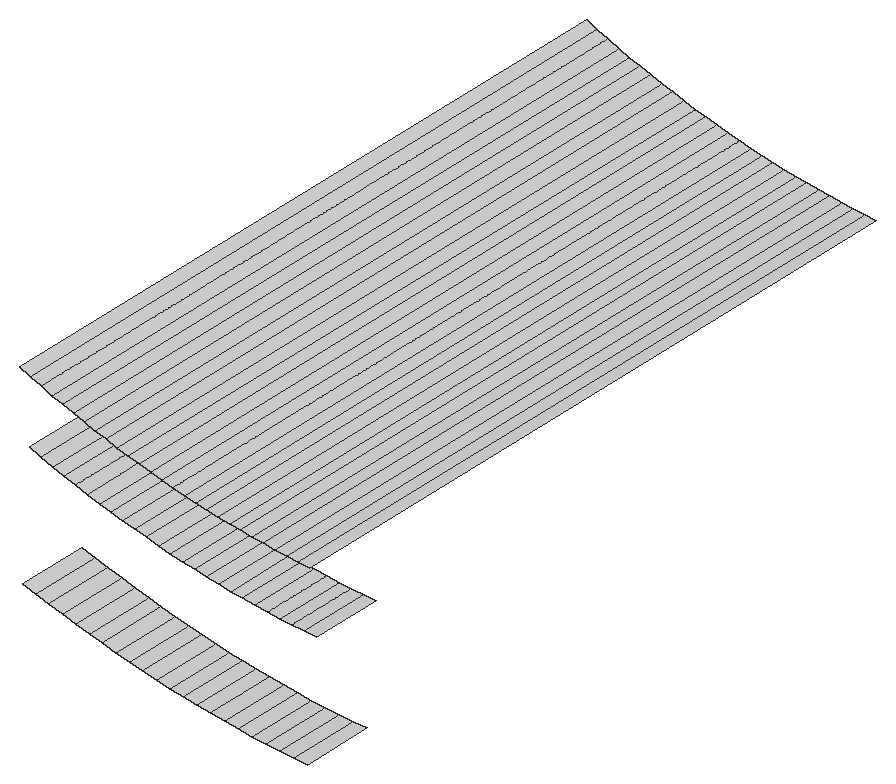
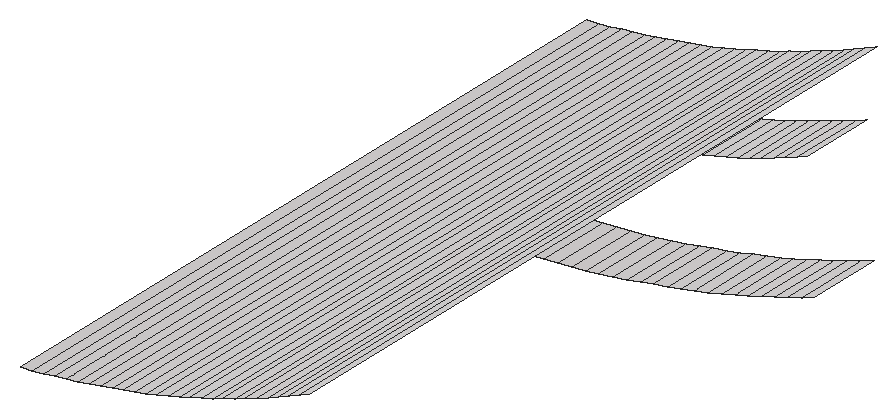
# SketchUp Ruby script. Lengths in inches.
U = 1.inch
M = Sketchup.active_model
def pt(a) = Geom::Point3d.new(a.map { |v| v * U })
def face(e, loops, mat)
  f = e.add_face(loops[0].map { |a| pt(a) })
  loops[1..].each { |l| e.add_face(l.map { |a| pt(a) }).erase! }
  f.material = f.back_material = mat if mat
  f
end
# faces: each face lists its corners as indices into pts; further lists are holes
def faces(e, pts, list, mat = nil) = list.each { |f| face(e, (f[0].is_a?(Array) ? f : [f]).map { |l| l.map { |i| pts[i] } }, mat) }
# xy, xz, yz: faces in a plane at the given z, y or x. An outline is a flat list of corners, or four numbers for a rectangle; further outlines are holes
def ring(l) = l.size == 4 ? [[l[0], l[1]], [l[2], l[1]], [l[2], l[3]], [l[0], l[3]]] : l.each_slice(2).to_a
def flat(e, list, mat, &to3) = list.each { |f| face(e, (f[0].is_a?(Array) ? f : [f]).map { |l| ring(l).map { |u, v| to3.(u, v) } }, mat) }
def xy(e, z, list, mat = nil) = flat(e, list, mat) { |x, y| [x, y, z] }
def xz(e, y, list, mat = nil) = flat(e, list, mat) { |x, z| [x, y, z] }
def yz(e, x, list, mat = nil) = flat(e, list, mat) { |y, z| [x, y, z] }
def lines(e, pts, list) = list.each { |a, b| e.add_line(pt(pts[a]), pt(pts[b])) }
# prism: a flat outline (further loops are holes) pulled along v
def prism(e, loops, v, mat = nil)
  f = face(e, loops, mat); d = Geom::Vector3d.new(v.map { |x| x * U })
  f.pushpull(f.normal.samedirection?(d) ? d.length : -d.length)
end
def box(e, o, s, mat = nil) = prism(e, [[o, [o[0] + s[0], o[1], o[2]], [o[0] + s[0], o[1] + s[1], o[2]], [o[0], o[1] + s[1], o[2]]]], [0, 0, s[2]], mat)
def at(x, y, z, deg = 0) = Geom::Transformation.translation(pt([x, y, z])) * Geom::Transformation.rotation(ORIGIN, Z_AXIS, deg.degrees)
def axes(o, x, y, z) = Geom::Transformation.new([*x, 0, *y, 0, *z, 0, *pt(o).to_a, 1])
def part(name) = M.definitions.add(name)
# library, detail: a bought-in or finely detailed component or shape, given as its bounding box
def library(name, o, s) = part(name).tap { |d| box(d.entities, o, s) }
def detail(e, o, s) = box(e.add_group.entities, o, s)
def put(e, d, t, mat = nil) = e.add_instance(d, t).tap { |i| i.material = mat if mat }
def group(e, t, mat = nil) = e.add_group.tap { |g| g.transformation = t; g.material = mat if mat }.entities
root = M.entities
M.materials.add("[Quartz Light Brown]").color = [215, 212, 212]
p = [[291.15,144.25,150.15],[291.15,143,150.15],[291.38,143,150.125],[291.38,144.25,150.125],[291.62,143,150.1],[291.62,144.25,150.1],
  [291.85,143,150.08],[291.85,144.25,150.08],[292.09,143,150.06],[292.09,144.25,150.06],[290.45,144.25,150.26],[290.45,143,150.26],
  [290.68,143,150.22],[290.68,144.25,150.22],[290.92,143,150.1875],[290.92,144.25,150.1875],[289.76,144.25,150.39],[289.76,143,150.39],
  [289.99,143,150.35],[289.99,144.25,150.35],[290.22,143,150.3],[290.22,144.25,150.3],[289.3,144.25,150.5],[289.3,143,150.5],
  [289.53,143,150.44],[289.53,144.25,150.44],[289.07,144.25,150.55],[289.07,143,150.55],[288.61,144.25,150.68],[288.61,143,150.68],
  [288.84,143,150.61],[288.84,144.25,150.61],[288.16,144.25,150.81],[288.16,143,150.81],[288.39,143,150.74],[288.39,144.25,150.74],
  [287.9375,144.25,150.88],[287.9375,143,150.88],[287.71,144.25,150.96],[287.71,143,150.96],[287.27,144.25,151.11],[287.27,143,151.11],
  [287.49,143,151.03],[287.49,144.25,151.03],[292.24,143,152.05],[292.04,143,152.07],[292.04,144.25,152.07],[292.24,144.25,152.05],
  [291.41,143,152.14],[291.2,143,152.17],[291.2,144.25,152.17],[291.41,144.25,152.14],[291.62,143,152.11],[291.62,144.25,152.11],
  [291.83,143,152.09],[291.83,144.25,152.09],[290.79,143,152.23],[290.58,143,152.27],[290.58,144.25,152.27],[290.79,144.25,152.23],
  [291,143,152.2],[291,144.25,152.2],[290.17,143,152.35],[289.97,143,152.39],[289.97,144.25,152.39],[290.17,144.25,152.35],
  [290.38,143,152.31],[290.38,144.25,152.31],[289.76,143,152.44],[289.5625,143,152.49],[289.5625,144.25,152.49],[289.76,144.25,152.44],
  [289.36,143,152.55],[289.16,143,152.6],[289.16,144.25,152.6],[289.36,144.25,152.55],[288.96,143,152.66],[288.96,144.25,152.66],
  [288.76,143,152.72],[288.56,143,152.78],[288.56,144.25,152.78],[288.76,144.25,152.72],[288.36,143,152.85],[288.16,143,152.92],
  [288.16,144.25,152.92],[288.36,144.25,152.85],[287.96,143,152.99],[287.96,144.25,152.99],[287.77,143,153.0625],[287.77,144.25,153.0625],
  [287.57,143,153.14],[287.38,143,153.22],[287.38,144.25,153.22],[287.57,144.25,153.14],[291.35,143,153.16],[291.54,143,153.13],
  [291.54,155,153.13],[291.35,155,153.16],[291.74,143,153.1],[291.74,155,153.1],[291.93,143,153.08],[291.93,155,153.08],
  [292.13,143,153.0625],[292.13,155,153.0625],[290.77,143,153.25],[290.96,143,153.22],[290.96,155,153.22],[290.77,155,153.25],
  [291.15,143,153.18],[291.15,155,153.18],[290.19,143,153.37],[290.38,143,153.33],[290.38,155,153.33],[290.19,155,153.37],
  [290.57,143,153.29],[290.57,155,153.29],[289.81,143,153.46],[290,143,153.41],[290,155,153.41],[289.81,155,153.46],
  [289.43,143,153.5625],[289.62,143,153.51],[289.62,155,153.51],[289.43,155,153.5625],[289.05,143,153.67],[289.24,143,153.62],
  [289.24,155,153.62],[289.05,155,153.67],[288.68,143,153.8],[288.86,143,153.73],[288.86,155,153.73],[288.68,155,153.8],
  [288.49,143,153.86],[288.49,155,153.86],[288.125,143,154],[288.31,143,153.93],[288.31,155,153.93],[288.125,155,154],
  [287.94,143,154.07],[287.94,155,154.07],[287.58,143,154.22],[287.76,143,154.14],[287.76,155,154.14],[287.58,155,154.22],
  [287.4,143,154.3],[287.4,155,154.3],[287.22,143,154.38],[287.22,155,154.38]]
faces(root,p,[[0,1,2,3],[3,2,4,5],[5,4,6,7],[7,6,8,9],[10,11,12,13],[13,12,14,15],[15,14,1,0],[16,17,18,19],
  [19,18,20,21],[21,20,11,10],[22,23,24,25],[25,24,17,16],[26,27,23,22],[28,29,30,31],[31,30,27,26],[32,33,34,35],
  [35,34,29,28],[36,37,33,32],[38,39,37,36],[40,41,42,43],[43,42,39,38],[44,45,46,47],[48,49,50,51],[52,48,51,53],
  [54,52,53,55],[45,54,55,46],[56,57,58,59],[60,56,59,61],[49,60,61,50],[62,63,64,65],[66,62,65,67],[57,66,67,58],
  [68,69,70,71],[63,68,71,64],[72,73,74,75],[69,72,75,70],[73,76,77,74],[78,79,80,81],[76,78,81,77],[82,83,84,85],
  [79,82,85,80],[83,86,87,84],[86,88,89,87],[90,91,92,93],[88,90,93,89],[94,95,96,97],[95,98,99,96],[98,100,101,99],
  [100,102,103,101],[104,105,106,107],[105,108,109,106],[108,94,97,109],[110,111,112,113],[111,114,115,112],[114,104,107,115],[116,117,118,119],
  [117,110,113,118],[120,121,122,123],[121,116,119,122],[124,125,126,127],[125,120,123,126],[128,129,130,131],[129,124,127,130],[132,128,131,133],
  [134,135,136,137],[135,132,133,136],[138,134,137,139],[140,141,142,143],[141,138,139,142],[144,140,143,145],[146,144,145,147]],"[Quartz Light Brown]")
